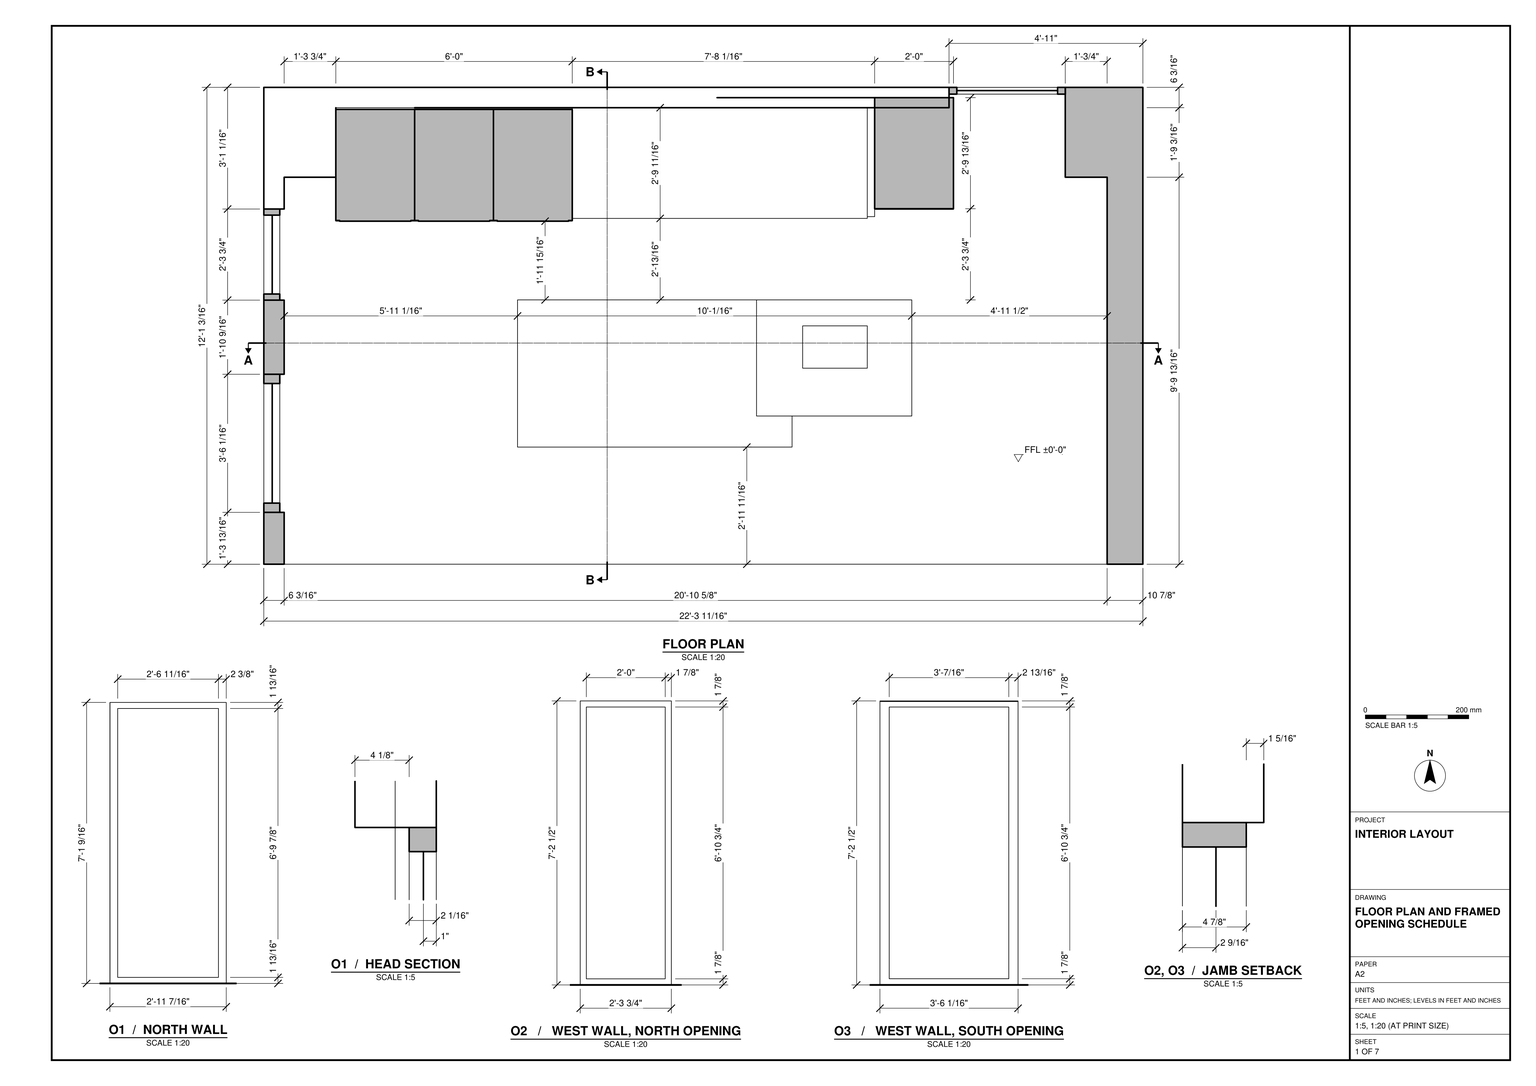
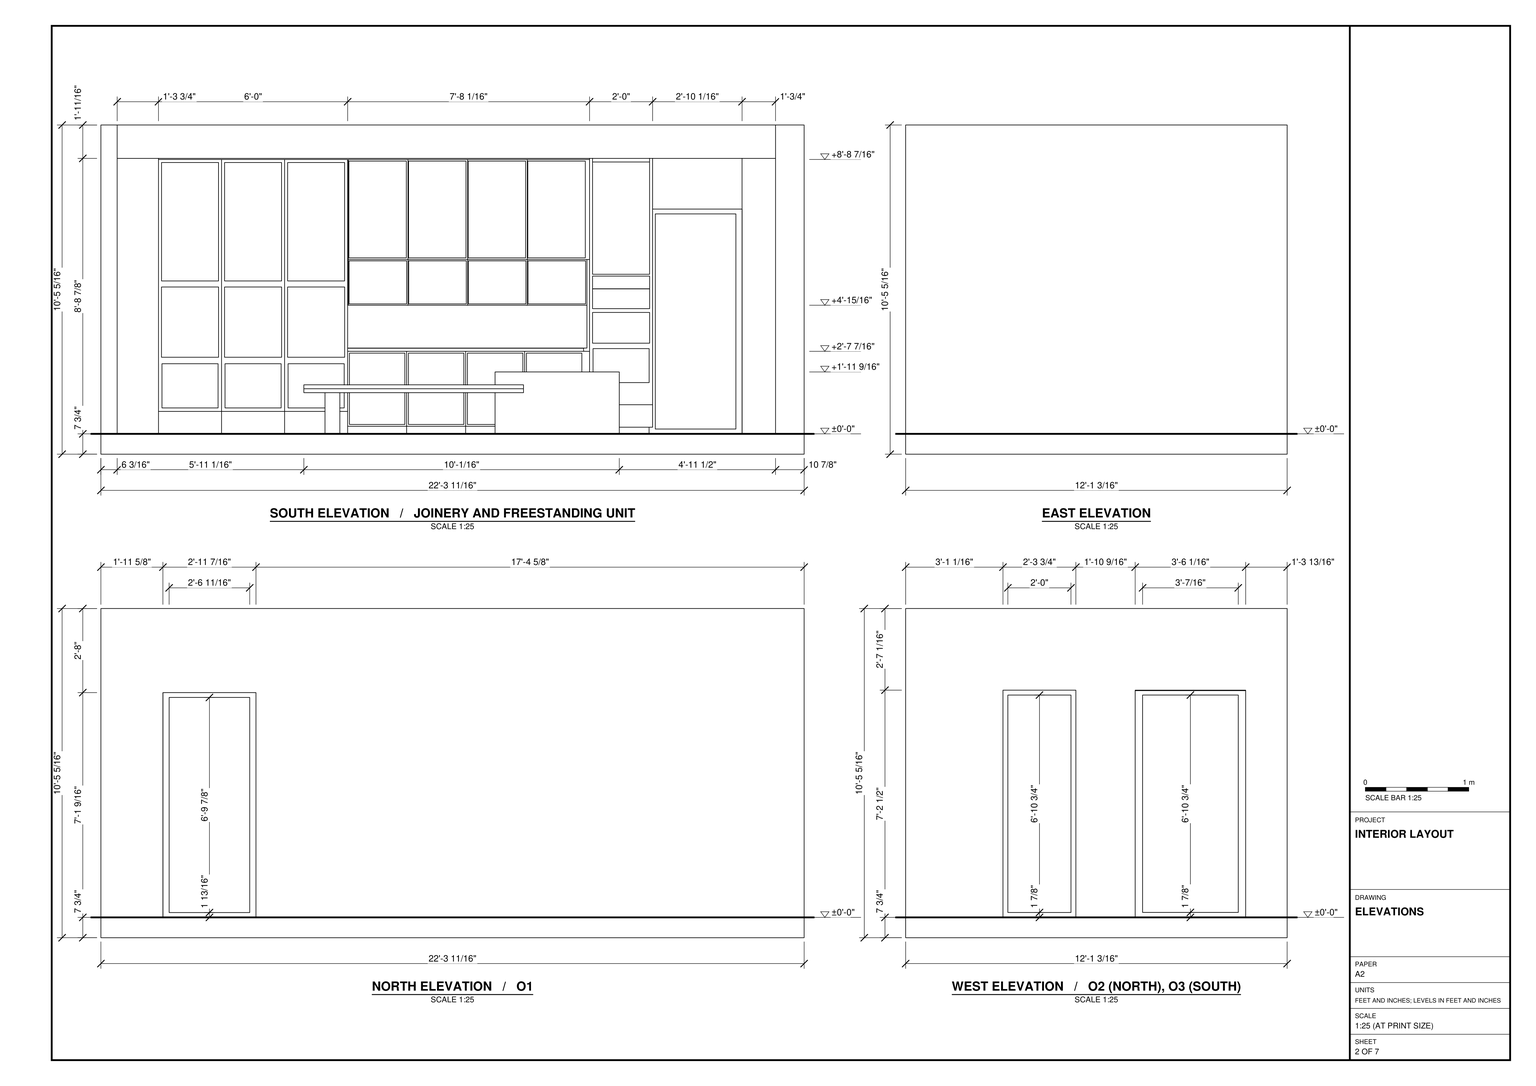
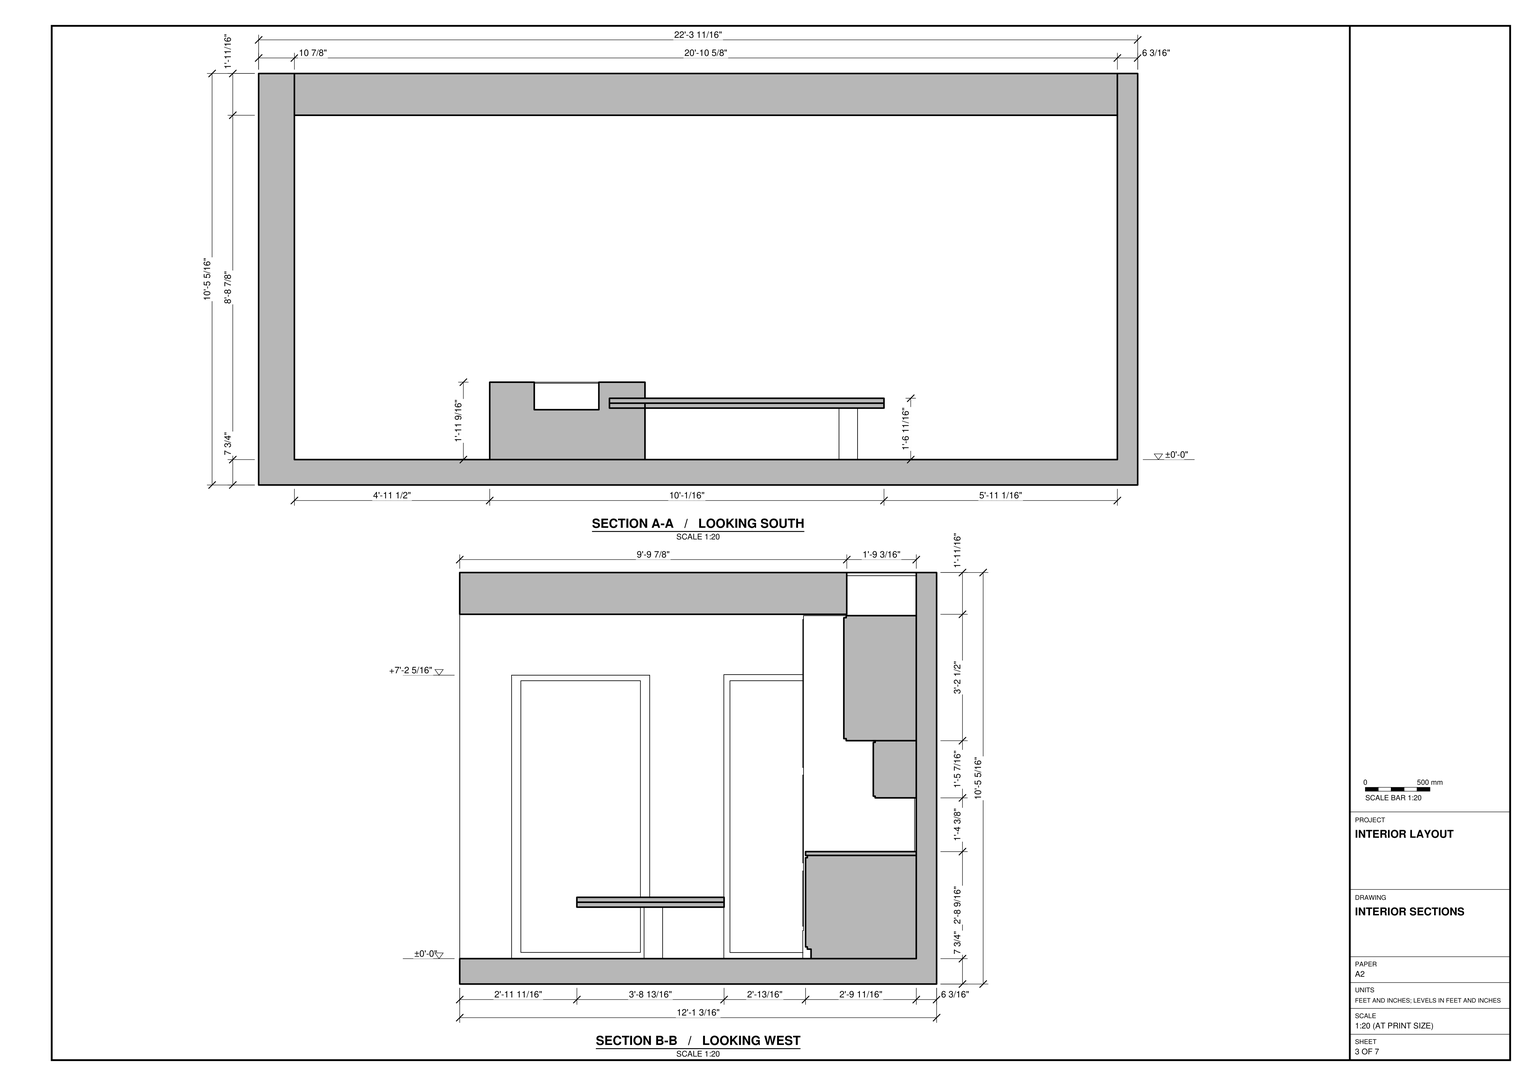
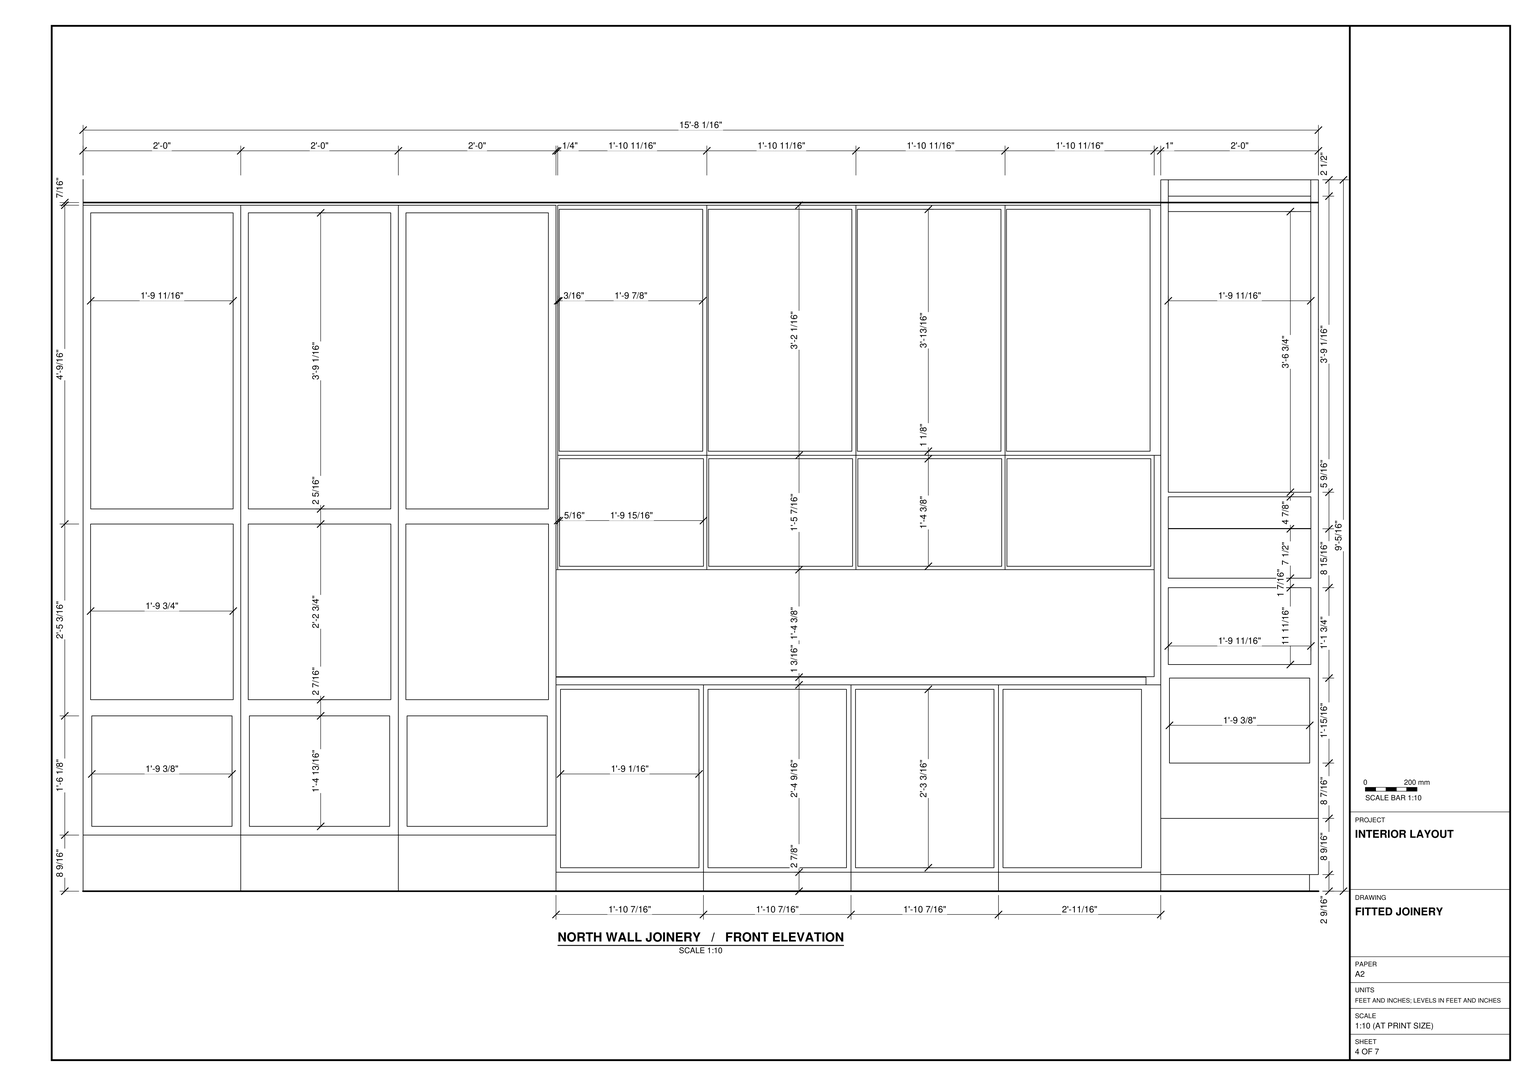
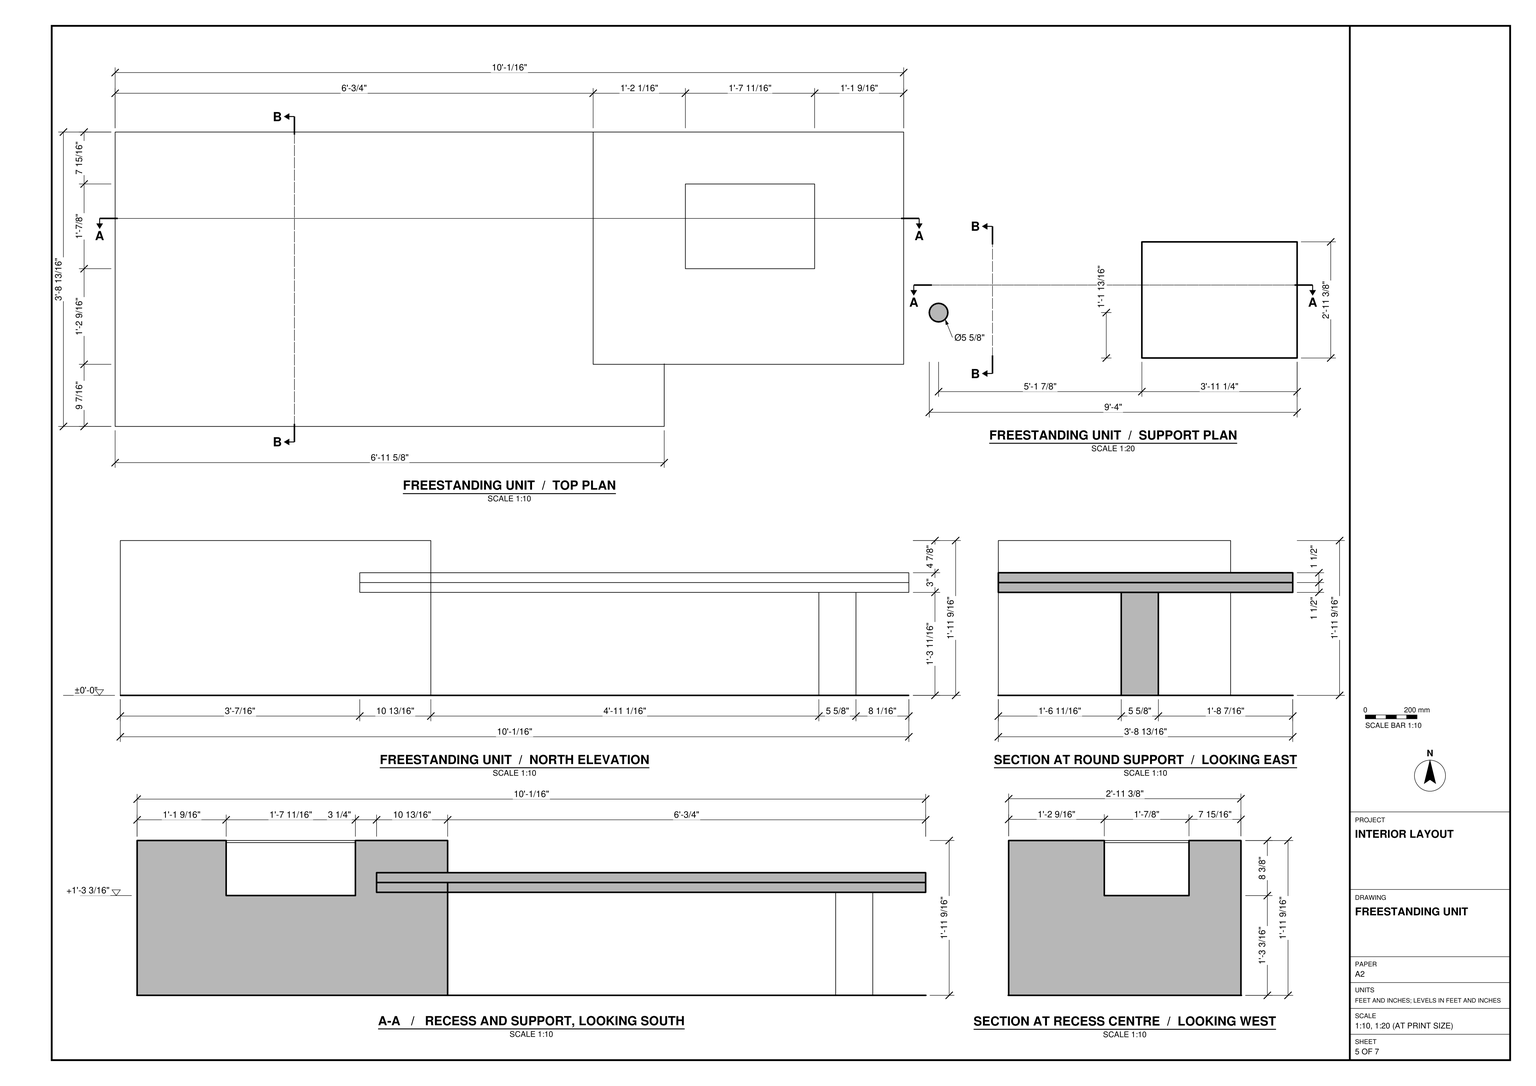
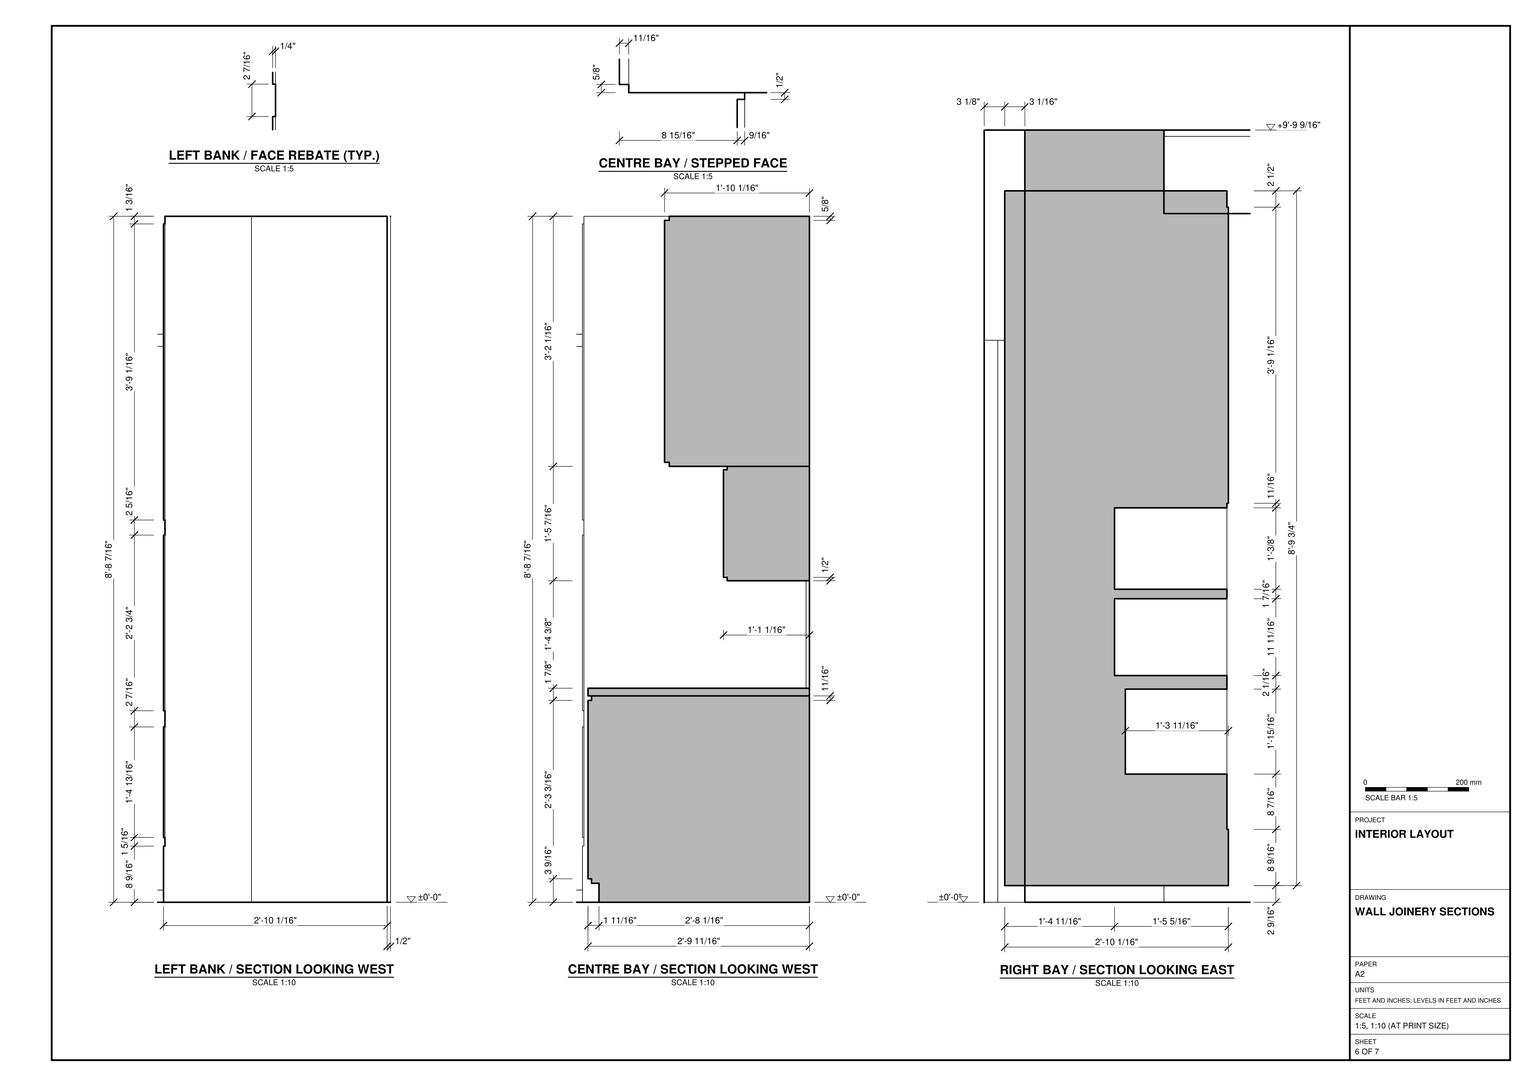
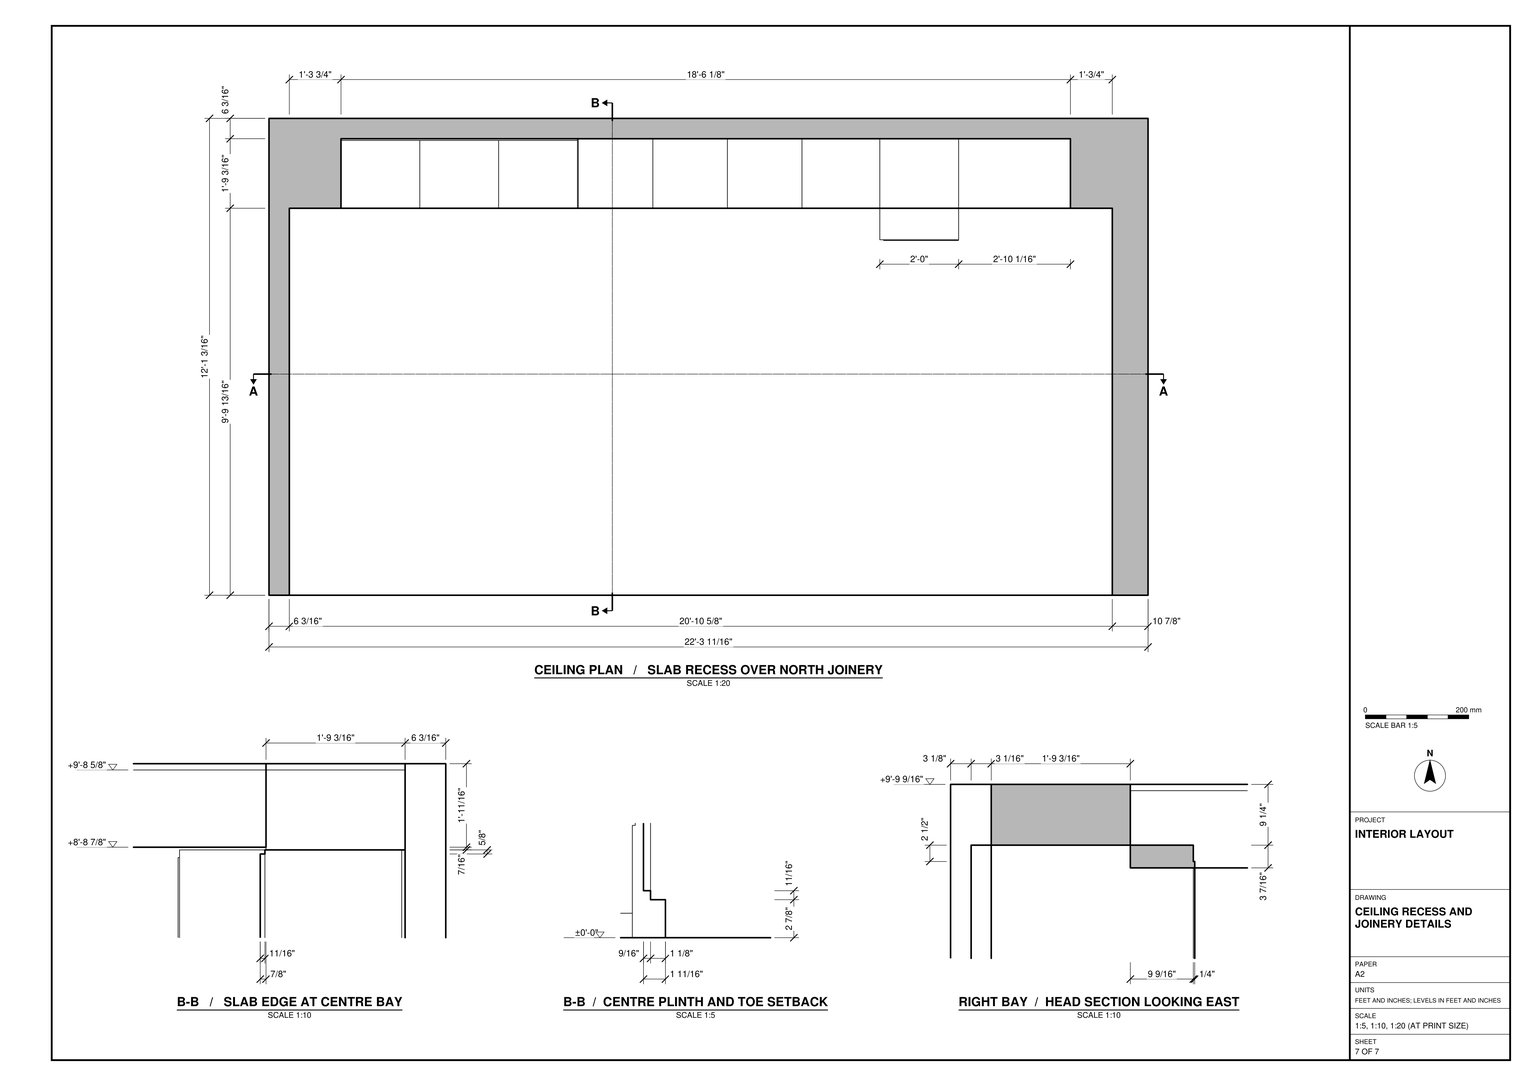
Work in feet and inches to model the interior shown in task_files/diagram_01.pdf. The room measures 22'-3 11/16" east to west, 12'-1 3/16" north to south and 10'-5 5/16" in overall height. Use the single finished floor level of ±0'-0"; measure the overall height from the underside of the floor slab, not from the finished floor.

Build the floor slab, walls and overhead shell members shown in section, leaving the south side open as drawn. Follow the wall thicknesses in plan, including the thicker return at the northeast corner. Form the framed opening near the east end of the north wall and the two unequal framed openings in the west wall. Use the opening schedule and sections to set the frames within the wall thickness.

Along the north wall, model the tall panelled cabinet bays, the central counter with base and upper cabinets, and the narrow storage unit beside the opening. Match the changes in cabinet depth and leave the space above the counter open. Position the freestanding unit using the plan clearances. Its thin supported tabletop extends west from the higher block, which has a rectangular recess in its top.

Keep shell elements and individual furniture or joinery pieces in separate groups or components, and use components for repeated parts. Any decor or loose items shown may use suitable library components. Save one SketchUp model as output_files/room_with_fitted_cabinetry_and_a_central_table_assembly.skp.

# SketchUp Ruby script. Lengths in inches.
U = 1.inch
M = Sketchup.active_model
def pt(a) = Geom::Point3d.new(a.map { |v| v * U })
def face(e, loops, mat)
  f = e.add_face(loops[0].map { |a| pt(a) })
  loops[1..].each { |l| e.add_face(l.map { |a| pt(a) }).erase! }
  f.material = f.back_material = mat if mat
  f
end
# faces: each face lists its corners as indices into pts; further lists are holes
def faces(e, pts, list, mat = nil) = list.each { |f| face(e, (f[0].is_a?(Array) ? f : [f]).map { |l| l.map { |i| pts[i] } }, mat) }
# xy, xz, yz: faces in a plane at the given z, y or x. An outline is a flat list of corners, or four numbers for a rectangle; further outlines are holes
def ring(l) = l.size == 4 ? [[l[0], l[1]], [l[2], l[1]], [l[2], l[3]], [l[0], l[3]]] : l.each_slice(2).to_a
def flat(e, list, mat, &to3) = list.each { |f| face(e, (f[0].is_a?(Array) ? f : [f]).map { |l| ring(l).map { |u, v| to3.(u, v) } }, mat) }
def xy(e, z, list, mat = nil) = flat(e, list, mat) { |x, y| [x, y, z] }
def xz(e, y, list, mat = nil) = flat(e, list, mat) { |x, z| [x, y, z] }
def yz(e, x, list, mat = nil) = flat(e, list, mat) { |y, z| [x, y, z] }
def lines(e, pts, list) = list.each { |a, b| e.add_line(pt(pts[a]), pt(pts[b])) }
# prism: a flat outline (further loops are holes) pulled along v
def prism(e, loops, v, mat = nil)
  f = face(e, loops, mat); d = Geom::Vector3d.new(v.map { |x| x * U })
  f.pushpull(f.normal.samedirection?(d) ? d.length : -d.length)
end
def box(e, o, s, mat = nil) = prism(e, [[o, [o[0] + s[0], o[1], o[2]], [o[0] + s[0], o[1] + s[1], o[2]], [o[0], o[1] + s[1], o[2]]]], [0, 0, s[2]], mat)
def at(x, y, z, deg = 0) = Geom::Transformation.translation(pt([x, y, z])) * Geom::Transformation.rotation(ORIGIN, Z_AXIS, deg.degrees)
def axes(o, x, y, z) = Geom::Transformation.new([*x, 0, *y, 0, *z, 0, *pt(o).to_a, 1])
def part(name) = M.definitions.add(name)
# library, detail: a bought-in or finely detailed component or shape, given as its bounding box
def library(name, o, s) = part(name).tap { |d| box(d.entities, o, s) }
def detail(e, o, s) = box(e.add_group.entities, o, s)
def put(e, d, t, mat = nil) = e.add_instance(d, t).tap { |i| i.material = mat if mat }
def group(e, t, mat = nil) = e.add_group.tap { |g| g.transformation = t; g.material = mat if mat }.entities
root = M.entities
M.materials.add("[Carrera Marble]").color = [207, 207, 207]
M.materials.add("[Color M05]").color = [114, 114, 114]
M.materials.add("[Tile Ceramic Natural]").color = [189, 180, 134]
M.materials.add("[Translucent Glass Gray]").color = [128, 128, 128]
M.materials["[Translucent Glass Gray]"].alpha = 0.5
M.materials.add("[Wood Bamboo]").color = [177, 105, 43]
M.materials.add("[Wood Veneer 02]").color = [190, 128, 91]
c1 = part("Group\#1")
xy(c1.entities,0,[[-4.86,0,0,27.75]])
xy(c1.entities,1.86,[[-4.86,1.86,-2.31,25.89],[-2.31,1.86,0,25.89]])
xy(c1.entities,84.64,[[-4.86,1.86,-2.31,25.89],[-2.31,1.86,0,25.89]])
xy(c1.entities,86.5,[[-4.86,0,0,27.75]])
xz(c1.entities,0,[[-4.86,0,0,86.5]])
xz(c1.entities,1.86,[[-4.86,1.86,-2.31,84.64],[-2.31,1.86,0,84.64]])
xz(c1.entities,25.89,[[-4.86,1.86,-2.31,84.64],[-2.31,1.86,0,84.64]])
xz(c1.entities,27.75,[[-4.86,0,0,86.5]])
yz(c1.entities,-4.86,[[[0,0,27.75,86.5],[1.86,1.86,25.89,84.64]]],"[Color M05]")
yz(c1.entities,-2.31,[[1.86,1.86,25.89,84.64]],"[Translucent Glass Gray]")
yz(c1.entities,0,[[[0,0,27.75,86.5],[1.86,1.86,25.89,84.64]]])
xy(root,0,[[0,0,267.67,145.21]])
xy(root,6.43,[[88.125,56.13,87.39,56.23,86.71,56.51,86.13,56.96,85.68,57.54,85.4,58.22,85.3,58.95,85.4,59.6875,85.68,60.37,86.13,60.95,86.71,61.4,87.39,61.68,88.125,61.78,88.86,61.68,89.54,61.4,90.125,60.95,90.57,60.37,90.86,59.6875,90.95,58.95,90.86,58.22,90.57,57.54,90.125,56.96,89.54,56.51,88.86,56.23]])
xy(root,7.74,[[6.19,0,256.79,0,256.79,117.84,244.04,117.84,244.04,145.21,208.65,145.21,208.65,139.02,21.92,139.02,21.92,117.84,6.19,117.84,6.19,108.17,0,108.17,0,80.42,6.19,80.42,6.19,57.84,0,57.84,0,15.79,6.19,15.79]])
xy(root,23.42,[[88.125,56.13,88.86,56.23,89.54,56.51,90.125,56.96,90.57,57.54,90.86,58.22,90.95,58.95,90.86,59.6875,90.57,60.37,90.125,60.95,89.54,61.4,88.86,61.68,88.125,61.78,87.39,61.68,86.71,61.4,86.13,60.95,85.68,60.37,85.4,59.6875,85.3,58.95,85.4,58.22,85.68,57.54,86.13,56.96,86.71,56.51,87.39,56.23]])
xy(root,39.16,[[93.92,105.3,183.75,105.84]])
xy(root,40.33,[[93.92,105.3,183.75,139.02]],"[Carrera Marble]")
xy(root,93.3,[[208.65,139.02,244.04,145.21]])
xy(root,94.05,[[0,15.79,6.19,57.84]])
xy(root,94.23,[[0,80.42,6.19,108.17]])
xy(root,112.59,[[6.19,0,256.79,117.84]])
xy(root,125.3125,[[0,0,6.19,5.29],[6.19,0,256.79,117.84],[256.79,0,267.67,5.29],[0,5.29,6.19,5.29,6.19,117.84,21.92,117.84,21.92,139.02,244.04,139.02,244.04,117.84,256.79,117.84,256.79,5.29,267.67,5.29,267.67,145.21,0,145.21],[21.92,117.84,244.04,139.02]])
xz(root,0,[[0,0,267.67,0,267.67,125.3125,256.79,125.3125,256.79,7.74,6.19,7.74,6.19,125.3125,0,125.3125],[6.19,112.59,256.79,125.3125]])
xz(root,15.79,[[0,7.74,6.19,94.05]])
xz(root,57.84,[[0,7.74,6.19,94.05]])
xz(root,80.42,[[0,7.74,6.19,94.23]])
xz(root,105.3,[[93.92,39.16,183.75,40.33]],"[Carrera Marble]")
xz(root,108.17,[[0,7.74,6.19,94.23]])
xz(root,117.84,[[6.19,7.74,21.92,112.59],[244.04,7.74,256.79,112.59],[6.19,112.59,21.92,124.35],[21.92,112.59,244.04,125.3125],[244.04,112.59,256.79,124.35],
  [6.19,124.35,21.92,125.3125],[244.04,124.35,256.79,125.3125]])
xz(root,139.02,[[[45.92,7.74,208.65,7.74,208.65,93.3,244.04,93.3,244.04,124.35,21.92,124.35,21.92,112.1875,45.92,112.1875],[93.92,40.4,184.99,56.7],[93.92,39.16,183.75,40.33]],[93.92,39.16,183.75,40.33],[21.92,124.35,244.04,125.3125]])
xz(root,139.02,[[93.92,40.4,184.99,56.7]],"[Tile Ceramic Natural]")
xz(root,145.21,[[[0,0,267.67,125.3125],[208.65,7.74,244.04,93.3]]])
yz(root,0,[[[0,0,145.21,125.3125],[15.79,7.74,57.84,94.05],[80.42,7.74,108.17,94.23]]])
yz(root,6.19,[[0,7.74,15.79,7.74,15.79,94.05,57.84,94.05,57.84,7.74,80.42,7.74,80.42,94.23,108.17,94.23,108.17,7.74,117.84,7.74,117.84,112.59,0,112.59],[0,112.59,117.84,124.35],[0,124.35,117.84,125.3125]])
yz(root,21.92,[[117.84,7.74,139.02,124.35],[117.84,124.35,139.02,125.3125]])
yz(root,93.92,[[105.3,39.16,139.02,40.33]])
yz(root,183.75,[[105.3,39.16,139.02,40.33]])
yz(root,208.65,[[139.02,7.74,145.21,93.3]])
yz(root,244.04,[[117.84,7.74,117.84,124.35,139.02,124.35,139.02,93.3,145.21,93.3,145.21,7.74],[117.84,124.35,139.02,125.3125]])
yz(root,256.79,[[0,7.74,117.84,112.59],[0,112.59,117.84,124.35],[0,124.35,117.84,125.3125]])
yz(root,267.67,[[0,0,145.21,125.3125]])
p = [[88.125,56.13,23.42],[87.39,56.23,23.42],[87.39,56.23,6.43],[88.125,56.13,6.43],[88.86,56.23,23.42],[88.86,56.23,6.43],
  [86.71,56.51,23.42],[86.71,56.51,6.43],[89.54,56.51,23.42],[89.54,56.51,6.43],[86.13,56.96,23.42],[86.13,56.96,6.43],
  [90.125,56.96,23.42],[90.125,56.96,6.43],[85.68,57.54,23.42],[85.68,57.54,6.43],[90.57,57.54,23.42],[90.57,57.54,6.43],
  [85.4,58.22,23.42],[85.4,58.22,6.43],[90.86,58.22,23.42],[90.86,58.22,6.43],[85.3,58.95,23.42],[85.3,58.95,6.43],
  [90.95,58.95,23.42],[90.95,58.95,6.43],[85.4,59.6875,23.42],[85.4,59.6875,6.43],[90.86,59.6875,23.42],[90.86,59.6875,6.43],
  [85.68,60.37,23.42],[85.68,60.37,6.43],[90.57,60.37,23.42],[90.57,60.37,6.43],[86.13,60.95,23.42],[86.13,60.95,6.43],
  [90.125,60.95,23.42],[90.125,60.95,6.43],[86.71,61.4,23.42],[86.71,61.4,6.43],[89.54,61.4,23.42],[89.54,61.4,6.43],
  [87.39,61.68,23.42],[87.39,61.68,6.43],[88.86,61.68,23.42],[88.86,61.68,6.43],[88.125,61.78,23.42],[88.125,61.78,6.43],
  [186.13,130.32,60.43],[207.85,130.32,60.43],[186.13,130.32,60.38],[207.85,130.32,60.38],[164.07,72.58,30.99],[183.75,72.58,30.99],
  [183.75,59.6875,30.99],[164.07,59.6875,30.99],[187.15,108.03,112.59],[207.93,108.03,112.59],[209.97,108.03,112.59],[187.15,108.03,111.22],
  [207.93,108.03,111.22],[208.84,108.03,111.22]]
faces(root,p,[[0,1,2,3],[4,0,3,5],[1,6,7,2],[8,4,5,9],[6,10,11,7],[12,8,9,13],[10,14,15,11],[16,12,13,17],
  [14,18,19,15],[20,16,17,21],[18,22,23,19],[24,20,21,25],[22,26,27,23],[28,24,25,29],[26,30,31,27],[32,28,29,33],
  [30,34,35,31],[36,32,33,37],[34,38,39,35],[40,36,37,41],[38,42,43,39],[44,40,41,45],[42,46,47,43],[46,44,45,47]],"[Wood Bamboo]")
lines(root,p,[[48,49],[50,51],[52,53],[53,54],[54,55],[55,52],[56,57],[57,58],[59,60],[60,61]])
put(root,c1,at(4.86,80.42,7.74))
put(root,c1,axes([4.86,15.79,7.77],[1,0,0],[0,1.51574,0],[0,0,0.9996]))
put(root,c1,axes([244.07,145.21,7.74],[0,0.42501,0],[-1.2768,0,0],[0,0,0.98926]))
g1 = group(root,at(93.92,105.01,7.74),"[Color M05]")
g2 = group(g1,at(0,0.3,0))
xy(g2,0,[[0,1.67,22.46,33.71],[22.46,1.67,44.91,33.71],[44.91,1.67,67.37,33.71],[67.37,1.67,92.08,33.71]])
xy(g2,2.89,[[0,0.54,22.46,1.67],[22.46,0.54,44.91,1.67],[44.91,0.54,67.37,1.67],[67.37,0.54,92.08,1.67]])
xy(g2,3.58,[[0.6875,0,21.77,0.54],[23.14,0,44.23,0.54],[45.6,0,66.68,0.54],[68.06,0,89.14,0.54]])
xy(g2,30.74,[[0.6875,0,21.77,0.54],[23.14,0,44.23,0.54],[45.6,0,66.68,0.54],[68.06,0,89.14,0.54]])
xy(g2,31.43,[[0,0.54,22.46,33.71],[22.46,0.54,44.91,33.71],[44.91,0.54,67.37,33.71],[67.37,0.54,92.08,33.71]])
xz(g2,0,[[0.6875,3.58,21.77,30.74],[23.14,3.58,44.23,30.74],[45.6,3.58,66.68,30.74],[68.06,3.58,89.14,30.74]])
xz(g2,0.54,[[[0,2.89,22.46,31.43],[0.6875,3.58,21.77,30.74]],[[22.46,2.89,44.91,31.43],[23.14,3.58,44.23,30.74]],[[44.91,2.89,67.37,31.43],[45.6,3.58,66.68,30.74]],[[67.37,2.89,92.08,31.43],[68.06,3.58,89.14,30.74]]])
xz(g2,1.67,[[0,0,22.46,2.89],[22.46,0,44.91,2.89],[44.91,0,67.37,2.89],[67.37,0,92.08,2.89]])
xz(g2,33.71,[[0,0,22.46,31.43],[22.46,0,44.91,31.43],[44.91,0,67.37,31.43],[67.37,0,92.08,31.43]])
yz(g2,0,[[1.67,0,1.67,2.89,0.54,2.89,0.54,31.43,33.71,31.43,33.71,0]])
yz(g2,0.6875,[[0,3.58,0.54,30.74]])
yz(g2,21.77,[[0,3.58,0.54,30.74]])
yz(g2,22.46,[[1.67,0,1.67,2.89,0.54,2.89,0.54,31.43,33.71,31.43,33.71,0]])
yz(g2,23.14,[[0,3.58,0.54,30.74]])
yz(g2,44.23,[[0,3.58,0.54,30.74]])
yz(g2,44.91,[[1.67,0,1.67,2.89,0.54,2.89,0.54,31.43,33.71,31.43,33.71,0]])
yz(g2,45.6,[[0,3.58,0.54,30.74]])
yz(g2,66.68,[[0,3.58,0.54,30.74]])
yz(g2,67.37,[[1.67,0,1.67,2.89,0.54,2.89,0.54,31.43,33.71,31.43,33.71,0]])
yz(g2,68.06,[[0,3.58,0.54,30.74]])
yz(g2,89.14,[[0,3.58,0.54,30.74]])
yz(g2,92.08,[[1.67,0,33.71,0,33.71,31.43,0.54,31.43,0.54,2.89,1.67,2.89]])
g3 = group(root,at(161.29,139.02,56.7),"[Color M05]")
xy(g3,0,[[-67.11,-12.52,-44.41,0],[-44.41,-12.52,-21.7,0],[-21.7,-12.52,1,0],[1,-12.52,23.7,0]])
xy(g3,0.51,[[-66.83,-13.09,-44.92,-12.52],[-44.12,-13.09,-22.22,-12.52],[-21.42,-13.09,0.49,-12.52],[1.29,-13.09,23.19,-12.52]])
xy(g3,16.9,[[-66.83,-13.09,-44.92,-12.52],[-44.12,-13.09,-22.22,-12.52],[-21.42,-13.09,0.49,-12.52],[1.29,-13.09,23.19,-12.52]])
xy(g3,17.41,[[-67.11,-21.34,-44.41,-12.52],[-44.41,-21.34,-21.7,-12.52],[-21.7,-21.34,1,-12.52],[1,-21.34,24.71,-12.52],[-67.11,-12.52,-44.41,0],
  [-44.41,-12.52,-21.7,0],[-21.7,-12.52,1,0],[1,-12.52,23.7,0],[23.7,-12.52,24.71,0]])
xy(g3,18.03,[[-66.9,-22.06,-45.03,-21.34],[-44.19,-22.06,-22.33,-21.34],[-21.49,-22.06,0.375,-21.34],[1.21,-22.06,23.08,-21.34]])
xy(g3,54.87,[[-66.9,-22.06,-45.03,-21.34],[-44.19,-22.06,-22.33,-21.34],[-21.49,-22.06,0.375,-21.34],[1.21,-22.06,23.08,-21.34]])
xy(g3,55.49,[[-67.11,-21.34,-44.41,0],[-44.41,-21.34,-21.7,0],[-21.7,-21.34,1,0],[1,-21.34,24.71,0]])
xz(g3,-22.06,[[-66.9,18.03,-45.03,54.87],[-44.19,18.03,-22.33,54.87],[-21.49,18.03,0.375,54.87],[1.21,18.03,23.08,54.87]],"[Color M05]")
xz(g3,-21.34,[[[-67.11,17.41,-44.41,55.49],[-66.9,18.03,-45.03,54.87]],[[-44.41,17.41,-21.7,55.49],[-44.19,18.03,-22.33,54.87]],[[-21.7,17.41,1,55.49],[-21.49,18.03,0.375,54.87]],[[1,17.41,24.71,55.49],[1.21,18.03,23.08,54.87]]])
xz(g3,-13.09,[[-66.83,0.51,-44.92,16.9],[-44.12,0.51,-22.22,16.9],[-21.42,0.51,0.49,16.9],[1.29,0.51,23.19,16.9]],"[Wood Veneer 02]")
xz(g3,-12.52,[[[-67.11,0,-44.41,17.41],[-66.83,0.51,-44.92,16.9]],[[-44.41,0,-21.7,17.41],[-44.12,0.51,-22.22,16.9]],[[-21.7,0,1,17.41],[-21.42,0.51,0.49,16.9]],[[1,0,23.7,17.41],[1.29,0.51,23.19,16.9]]])
xz(g3,0,[[-67.11,0,-44.41,17.41],[-44.41,0,-21.7,17.41],[-21.7,0,1,17.41],[1,0,23.7,17.41],[-67.11,17.41,-44.41,55.49],
  [-44.41,17.41,-21.7,55.49],[-21.7,17.41,1,55.49],[1,17.41,24.71,55.49]])
yz(g3,-67.11,[[-12.52,0,0,17.41],[-21.34,17.41,0,55.49]])
yz(g3,-66.9,[[-22.06,18.03,-21.34,54.87]])
yz(g3,-66.83,[[-13.09,0.51,-12.52,16.9]])
yz(g3,-45.03,[[-22.06,18.03,-21.34,54.87]])
yz(g3,-44.92,[[-13.09,0.51,-12.52,16.9]])
yz(g3,-44.41,[[-12.52,0,0,17.41],[-21.34,17.41,0,55.49]])
yz(g3,-44.19,[[-22.06,18.03,-21.34,54.87]])
yz(g3,-44.12,[[-13.09,0.51,-12.52,16.9]])
yz(g3,-22.33,[[-22.06,18.03,-21.34,54.87]])
yz(g3,-22.22,[[-13.09,0.51,-12.52,16.9]])
yz(g3,-21.7,[[-12.52,0,0,17.41],[-21.34,17.41,0,55.49]])
yz(g3,-21.49,[[-22.06,18.03,-21.34,54.87]])
yz(g3,-21.42,[[-13.09,0.51,-12.52,16.9]])
yz(g3,0.375,[[-22.06,18.03,-21.34,54.87]])
yz(g3,0.49,[[-13.09,0.51,-12.52,16.9]])
yz(g3,1,[[-12.52,0,0,17.41],[-21.34,17.41,0,55.49]])
yz(g3,1.21,[[-22.06,18.03,-21.34,54.87]])
yz(g3,1.29,[[-13.09,0.51,-12.52,16.9]])
yz(g3,23.08,[[-22.06,18.03,-21.34,54.87]])
yz(g3,23.19,[[-13.09,0.51,-12.52,16.9]])
yz(g3,23.7,[[-12.52,0,0,17.41]])
yz(g3,24.71,[[-21.34,17.41,0,55.49]])
g4 = group(root,at(150.03,45.125,7.74),"[Carrera Marble]")
g5 = group(g4,at(0,0,0))
xy(g5,0,[[0,0,47.28,35.37]])
xy(g5,15.19,[[14.04,14.5625,33.72,27.46]])
xy(g5,23.57,[[[0,0,47.28,35.37],[14.04,14.5625,33.72,27.46]]])
xz(g5,0,[[0,0,47.28,23.57]])
xz(g5,14.5625,[[14.04,15.19,33.72,23.57]])
xz(g5,27.46,[[14.04,15.19,33.72,23.57]])
xz(g5,35.37,[[0,0,47.28,23.57]])
yz(g5,0,[[0,0,35.37,17.18],[0,18.68,35.37,23.57]])
yz(g5,14.04,[[14.5625,15.19,27.46,23.57]])
yz(g5,33.72,[[14.5625,15.19,27.46,23.57]])
yz(g5,47.28,[[0,0,35.37,23.57]])
g6 = group(g5,at(0,0,17.18),"[Wood Bamboo]")
xy(g6,-1.5,[[-72.78,-9.46,10.82,35.37]])
xy(g6,0,[[-72.78,-9.46,10.82,35.37]])
xy(g6,1.5,[[-72.78,-9.46,10.82,35.37]])
xz(g6,-9.46,[[-72.78,-1.5,10.82,0],[-72.78,0,10.82,1.5]])
xz(g6,35.37,[[-72.78,-1.5,10.82,0],[-72.78,0,10.82,1.5]])
yz(g6,-72.78,[[-9.46,-1.5,35.37,0],[-9.46,0,35.37,1.5]])
yz(g6,10.82,[[-9.46,-1.5,35.37,0],[-9.46,0,35.37,1.5]])
g7 = group(root,at(21.92,135.77,7.74),"[Color M05]")
xy(g7,0,[[0,-31.3125,24,2.73],[24,-31.3125,48,2.73],[48,-31.3125,72,2.73]])
xy(g7,2.54,[[164.08,-27.74,188.08,6.31]])
xy(g7,8.55,[[0,-31.3125,24,-31.09],[24,-31.3125,48,-31.09],[48,-31.3125,72,-31.09]])
xy(g7,9.87,[[1.32,-31.3125,22.68,-31.09],[25.32,-31.3125,46.68,-31.09],[49.32,-31.3125,70.68,-31.09]])
xy(g7,11.09,[[164.08,-27.74,188.08,-27.52]])
xy(g7,19.51,[[165.4,-27.52,186.75,-12.05]])
xy(g7,26.7,[[1.32,-31.3125,22.68,-31.09],[25.32,-31.3125,46.68,-31.09],[49.32,-31.3125,70.68,-31.09]])
xy(g7,29.16,[[1.14,-31.3125,22.86,-31.09],[25.14,-31.3125,46.86,-31.09],[49.14,-31.3125,70.86,-31.09]])
xy(g7,32.46,[[165.4,-27.52,186.75,-12.05]])
xy(g7,34.52,[[165.22,-27.52,186.9375,-10.41]])
xy(g7,46.22,[[165.22,-27.52,186.9375,-10.41]])
xy(g7,47.66,[[165.22,-27.52,186.9375,-10.41]])
xy(g7,55.91,[[1.14,-31.3125,22.86,-31.09],[25.14,-31.3125,46.86,-31.09],[49.14,-31.3125,70.86,-31.09]])
xy(g7,58.21,[[1.16,-31.3125,22.84,-31.09],[25.16,-31.3125,46.84,-31.09],[49.16,-31.3125,70.84,-31.09]])
xy(g7,60.05,[[165.22,-27.52,186.9375,-10.41]])
xy(g7,60.75,[[165.23,-27.74,186.92,-27.52]])
xy(g7,103.29,[[1.16,-31.3125,22.84,-31.09],[25.16,-31.3125,46.84,-31.09],[49.16,-31.3125,70.84,-31.09]])
xy(g7,104.45,[[0,-31.09,24,2.73],[24,-31.09,48,2.73],[48,-31.09,72,2.73]])
xy(g7,105.83,[[165.23,-27.74,186.92,-27.52]])
xy(g7,108.32,[[164.08,-27.52,188.08,6.31]])
xz(g7,-31.3125,[[0,0,24,8.55],[24,0,48,8.55],[48,0,72,8.55],[1.32,9.87,22.68,26.7],[25.32,9.87,46.68,26.7],
  [49.32,9.87,70.68,26.7],[1.14,29.16,22.86,55.91],[25.14,29.16,46.86,55.91],[49.14,29.16,70.86,55.91],[1.16,58.21,22.84,103.29],
  [25.16,58.21,46.84,103.29],[49.16,58.21,70.84,103.29]])
xz(g7,-31.09,[[[0,8.55,24,104.45],[1.16,58.21,22.84,103.29],[1.14,29.16,22.86,55.91],[1.32,9.87,22.68,26.7]],[[24,8.55,48,104.45],[25.16,58.21,46.84,103.29],[25.14,29.16,46.86,55.91],[25.32,9.87,46.68,26.7]],[[48,8.55,72,104.45],[49.16,58.21,70.84,103.29],[49.14,29.16,70.86,55.91],[49.32,9.87,70.68,26.7]]])
xz(g7,-27.74,[[164.08,2.54,188.08,11.09],[165.23,60.75,186.92,105.83]])
xz(g7,-27.52,[[[164.08,11.09,188.08,11.09,188.08,108.32,186.92,108.32,186.92,60.75,165.23,60.75,165.23,108.32,164.08,108.32],[165.4,19.51,186.75,32.46],[165.22,47.66,186.9375,60.05],[165.22,34.52,186.9375,46.22]],[165.23,105.83,186.92,108.32]])
xz(g7,-12.05,[[165.4,19.51,186.75,32.46]])
xz(g7,-10.41,[[165.22,34.52,186.9375,46.22],[165.22,47.66,186.9375,55.1875],[165.22,55.1875,186.9375,55.23],[165.22,55.23,186.9375,60.05]])
xz(g7,2.73,[[0,0,24,104.45],[24,0,48,104.45],[48,0,72,104.45]])
xz(g7,6.31,[[116.08,2.54,164.08,106.99],[164.08,2.54,188.08,108.32]])
yz(g7,0,[[-31.3125,0,-31.3125,8.55,-31.09,8.55,-31.09,104.45,2.73,104.45,2.73,0]])
yz(g7,1.14,[[-31.3125,29.16,-31.09,55.91]])
yz(g7,1.16,[[-31.3125,58.21,-31.09,103.29]])
yz(g7,1.32,[[-31.3125,9.87,-31.09,26.7]])
yz(g7,22.68,[[-31.3125,9.87,-31.09,26.7]])
yz(g7,22.84,[[-31.3125,58.21,-31.09,103.29]])
yz(g7,22.86,[[-31.3125,29.16,-31.09,55.91]])
yz(g7,24,[[-31.3125,0,-31.3125,8.55,-31.09,8.55,-31.09,104.45,2.73,104.45,2.73,0]])
yz(g7,25.14,[[-31.3125,29.16,-31.09,55.91]])
yz(g7,25.16,[[-31.3125,58.21,-31.09,103.29]])
yz(g7,25.32,[[-31.3125,9.87,-31.09,26.7]])
yz(g7,46.68,[[-31.3125,9.87,-31.09,26.7]])
yz(g7,46.84,[[-31.3125,58.21,-31.09,103.29]])
yz(g7,46.86,[[-31.3125,29.16,-31.09,55.91]])
yz(g7,48,[[-31.3125,0,-31.3125,8.55,-31.09,8.55,-31.09,104.45,2.73,104.45,2.73,0]])
yz(g7,49.14,[[-31.3125,29.16,-31.09,55.91]])
yz(g7,49.16,[[-31.3125,58.21,-31.09,103.29]])
yz(g7,49.32,[[-31.3125,9.87,-31.09,26.7]])
yz(g7,70.68,[[-31.3125,9.87,-31.09,26.7]])
yz(g7,70.84,[[-31.3125,58.21,-31.09,103.29]])
yz(g7,70.86,[[-31.3125,29.16,-31.09,55.91]])
yz(g7,72,[[-31.3125,0,2.73,0,2.73,104.45,-31.09,104.45,-31.09,8.55,-31.3125,8.55]])
yz(g7,164.08,[[-27.74,2.54,-27.74,11.09,-27.52,11.09,-27.52,108.32,6.31,108.32,6.31,2.54]])
yz(g7,165.22,[[-27.52,34.52,-10.41,46.22],[-27.52,47.66,-10.41,60.05]])
yz(g7,165.23,[[-27.74,60.75,-27.52,105.83]])
yz(g7,165.4,[[-27.52,19.51,-12.05,32.46]])
yz(g7,186.75,[[-27.52,19.51,-12.05,32.46]])
yz(g7,186.92,[[-27.74,60.75,-27.52,105.83]])
yz(g7,186.9375,[[-27.52,34.52,-10.41,46.22],[-27.52,47.66,-10.41,60.05]])
yz(g7,188.08,[[-27.74,2.54,6.31,2.54,6.31,108.32,-27.52,108.32,-27.52,11.09,-27.74,11.09]])
p = [[139.07,-26.03,8.55],[139.07,-25.81,8.55],[140.21,-26.03,55.91],[140.21,-25.81,55.91],[140.21,-26.03,29.16],[140.21,-25.81,29.16],
  [161.93,-26.03,29.16],[161.93,-25.81,29.16],[161.93,-26.03,55.91],[161.93,-25.81,55.91],[140.23,-26.03,103.29],[140.23,-25.81,103.29],
  [140.23,-26.03,58.21],[140.23,-25.81,58.21],[161.75,-26.03,9.87],[161.75,-25.81,9.87],[161.75,-26.03,26.7],[161.75,-25.81,26.7],
  [161.92,-26.03,58.21],[161.92,-25.81,58.21],[161.92,-26.03,103.29],[161.92,-25.81,103.29],[140.4,-26.03,9.87],[140.4,-25.81,9.87],
  [140.4,-26.03,26.7],[140.4,-25.81,26.7],[116.4,-26.03,9.87],[116.4,-25.81,9.87],[116.4,-26.03,26.7],[116.4,-25.81,26.7],
  [137.92,-26.03,58.21],[137.92,-25.81,58.21],[137.75,-26.03,26.7],[137.75,-25.81,26.7],[116.21,-26.03,55.91],[116.21,-25.81,55.91],
  [116.21,-26.03,29.16],[116.21,-25.81,29.16],[137.75,-26.03,9.87],[137.75,-25.81,9.87],[115.07,-26.03,8.55],[115.07,-25.81,8.55],
  [137.92,-26.03,103.29],[137.92,-25.81,103.29],[116.23,-26.03,58.21],[116.23,-25.81,58.21],[116.23,-26.03,103.29],[116.23,-25.81,103.29],
  [137.93,-26.03,55.91],[137.93,-25.81,55.91],[137.93,-26.03,29.16],[137.93,-25.81,29.16]]
lines(g7,p,[[0,1],[2,3],[4,5],[6,7],[8,9],[10,11],[12,13],[14,15],[16,17],[18,19],[20,21],[22,23],
  [24,25],[26,27],[28,29],[30,31],[32,33],[34,35],[36,37],[38,39],[40,41],[42,43],[44,45],[46,47],
  [48,49],[50,51]])
